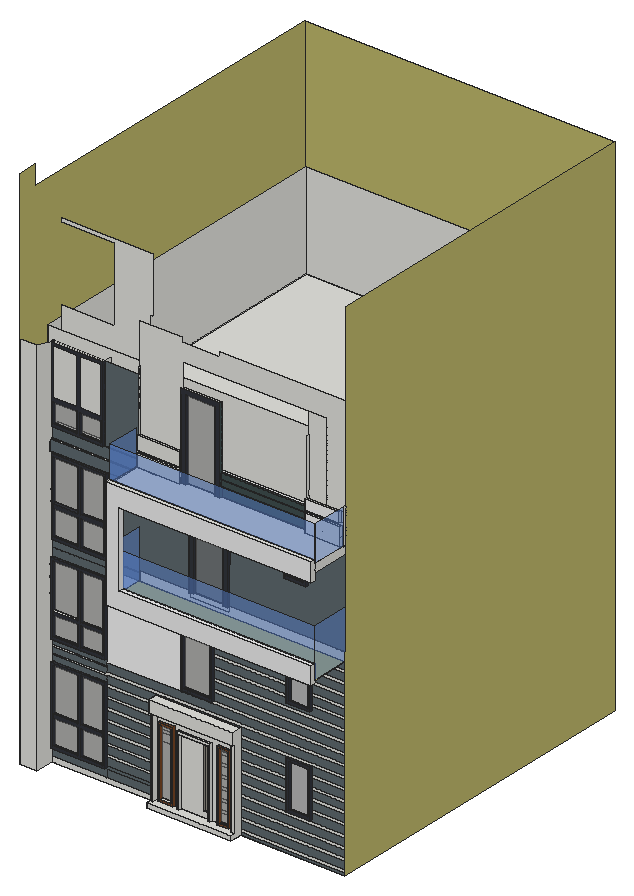
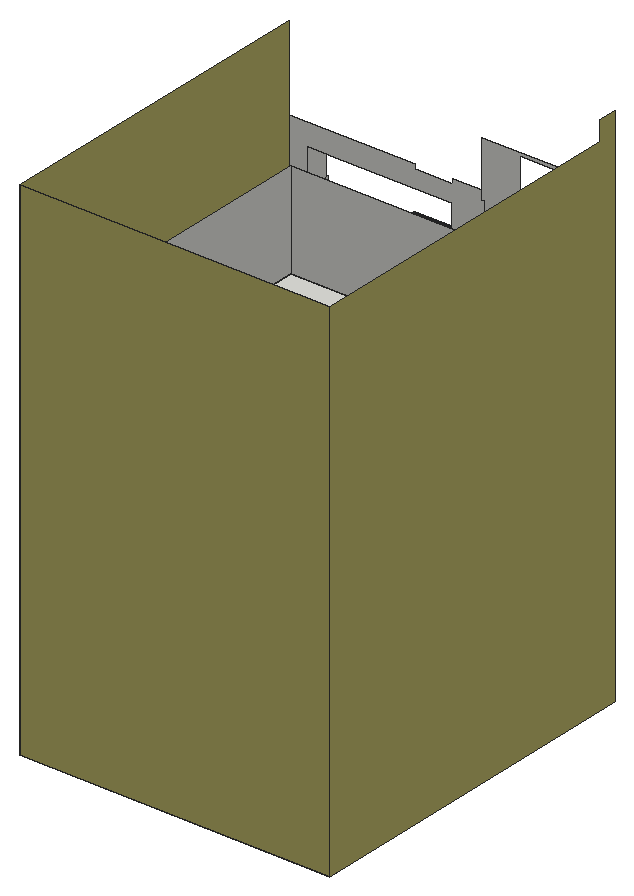
# SketchUp Ruby script. Lengths in inches.
U = 1.inch
M = Sketchup.active_model
def pt(a) = Geom::Point3d.new(a.map { |v| v * U })
def face(e, loops, mat)
  f = e.add_face(loops[0].map { |a| pt(a) })
  loops[1..].each { |l| e.add_face(l.map { |a| pt(a) }).erase! }
  f.material = f.back_material = mat if mat
  f
end
# faces: each face lists its corners as indices into pts; further lists are holes
def faces(e, pts, list, mat = nil) = list.each { |f| face(e, (f[0].is_a?(Array) ? f : [f]).map { |l| l.map { |i| pts[i] } }, mat) }
# xy, xz, yz: faces in a plane at the given z, y or x. An outline is a flat list of corners, or four numbers for a rectangle; further outlines are holes
def ring(l) = l.size == 4 ? [[l[0], l[1]], [l[2], l[1]], [l[2], l[3]], [l[0], l[3]]] : l.each_slice(2).to_a
def flat(e, list, mat, &to3) = list.each { |f| face(e, (f[0].is_a?(Array) ? f : [f]).map { |l| ring(l).map { |u, v| to3.(u, v) } }, mat) }
def xy(e, z, list, mat = nil) = flat(e, list, mat) { |x, y| [x, y, z] }
def xz(e, y, list, mat = nil) = flat(e, list, mat) { |x, z| [x, y, z] }
def yz(e, x, list, mat = nil) = flat(e, list, mat) { |y, z| [x, y, z] }
def lines(e, pts, list) = list.each { |a, b| e.add_line(pt(pts[a]), pt(pts[b])) }
# prism: a flat outline (further loops are holes) pulled along v
def prism(e, loops, v, mat = nil)
  f = face(e, loops, mat); d = Geom::Vector3d.new(v.map { |x| x * U })
  f.pushpull(f.normal.samedirection?(d) ? d.length : -d.length)
end
def box(e, o, s, mat = nil) = prism(e, [[o, [o[0] + s[0], o[1], o[2]], [o[0] + s[0], o[1] + s[1], o[2]], [o[0], o[1] + s[1], o[2]]]], [0, 0, s[2]], mat)
def at(x, y, z, deg = 0) = Geom::Transformation.translation(pt([x, y, z])) * Geom::Transformation.rotation(ORIGIN, Z_AXIS, deg.degrees)
def axes(o, x, y, z) = Geom::Transformation.new([*x, 0, *y, 0, *z, 0, *pt(o).to_a, 1])
def part(name) = M.definitions.add(name)
# library, detail: a bought-in or finely detailed component or shape, given as its bounding box
def library(name, o, s) = part(name).tap { |d| box(d.entities, o, s) }
def detail(e, o, s) = box(e.add_group.entities, o, s)
def put(e, d, t, mat = nil) = e.add_instance(d, t).tap { |i| i.material = mat if mat }
def group(e, t, mat = nil) = e.add_group.tap { |g| g.transformation = t; g.material = mat if mat }.entities
root = M.entities
M.materials.add("[0057_DarkKhaki]").color = [189, 183, 107]
M.materials.add("[0078_DarkSlateGray]").color = [63, 79, 79]
M.materials.add("[Black Pen 2]").color = [244, 244, 244]
M.materials.add("[Color M00]").color = [255, 255, 255]
M.materials.add("[Formica Graystone]").color = [149, 146, 135]
M.materials.add("[Formica Laminate Dark]").color = [50, 53, 60]
M.materials.add("[Formica Speckled Grey]").color = [94, 105, 111]
M.materials.add("[Mirror 01]").color = [185, 185, 185]
M.materials.add("[Stone Random Ashlar]").color = [240, 240, 240]
M.materials.add("[Translucent Glass Blue]").color = [100, 149, 237]
M.materials["[Translucent Glass Blue]"].alpha = 0.5
M.materials.add("[Translucent Glass Gray]").color = [128, 128, 128]
M.materials["[Translucent Glass Gray]"].alpha = 0.5
M.materials.add("[Windmill]").color = [236, 236, 236]
M.materials.add("[Wood Veneer 01]").color = [120, 70, 37]
xy(root,0,[[0,30,21.02,54],[150.64,39,255.96,51],[150.64,51,255.96,54],[[0,54,386.375,474.125],[9,63,377.375,465.125]],[9,63,377.375,465.125]])
xy(root,6.14,[[150.64,39,255.96,39,255.96,45,251.09,45,251.09,51,246.22,51,246.22,48,231.47,48,231.47,51,222.98,51,222.98,48,219.98,48,219.98,51,183.98,51,183.98,48,180.98,48,180.98,51,176.24,51,176.24,48,157.55,48,157.55,51,154.1,51,154.1,45,150.64,45],[157.55,48,176.24,51],[180.98,48,183.98,51],[219.98,48,222.98,51],[231.47,48,239.96,51],
  [239.96,48,246.22,51]])
xy(root,8.03,[[233.36,48,239.96,51],[239.96,48,244.33,51]])
xy(root,9.14,[[160.55,48,173.24,51]])
xy(root,13.03,[[212.45,51,217.33,53.3125]],"[Formica Graystone]")
xy(root,16.57,[[21.02,51,89.14,54]],"[Formica Laminate Dark]")
xy(root,19.57,[[24.02,51,55.08,54],[59.33,51,86.14,54]],"[Formica Laminate Dark]")
xy(root,48.67,[[315.34,51,344.65,54]])
xy(root,51.45,[[24.02,51,55.08,54],[59.33,51,86.14,54]],"[Formica Laminate Dark]")
xy(root,51.67,[[318.34,51,341.65,54]],"[Formica Laminate Dark]")
xy(root,55.1875,[[24.02,51,55.08,54],[59.33,51,86.14,54]],"[Formica Laminate Dark]")
xy(root,87.16,[[212.45,51,217.33,53.3125]],"[Formica Graystone]")
xy(root,90.14,[[183.98,48,219.98,51]])
xy(root,91.94,[[233.36,48,244.33,51]],"[Wood Veneer 01]")
xy(root,92.07,[[160.55,48,173.24,51]],"[Wood Veneer 01]")
xy(root,93.14,[[180.98,48,222.98,51]])
xy(root,93.82,[[231.47,48,246.22,51]],"[Wood Veneer 01]")
xy(root,95.07,[[157.55,48,176.24,51]],"[Wood Veneer 01]")
xy(root,104.875,[[150.64,42,150.64,45,154.1,45,154.1,51,251.09,51,251.09,45,255.96,45,255.96,42],[239.96,51,239.98,54]])
xy(root,105.98,[[318.34,51,341.65,54]])
xy(root,108.98,[[315.34,51,344.65,54]],"[Formica Laminate Dark]")
xy(root,109.86,[[24.02,51,55.08,54],[59.33,51,86.14,54]],"[Formica Laminate Dark]")
xy(root,112.86,[[21.02,51,89.14,54]],"[Formica Laminate Dark]")
xy(root,120,[[150.64,42,255.96,54],[9,63,377.375,465.125]])
xy(root,138.01,[[183.4,51,222.71,54]],"[Formica Laminate Dark]")
xy(root,138.82,[[21.02,51,89.14,54]],"[Formica Laminate Dark]")
xy(root,141.01,[[186.4,51,219.71,54]],"[Formica Laminate Dark]")
xy(root,141.82,[[24.02,51,55.08,54],[59.1,51,86.14,54]])
xy(root,166.59,[[24.02,51,55.08,54],[59.1,51,86.14,54]],"[Formica Laminate Dark]")
xy(root,169.86,[[24.02,51,55.08,54],[59.1,51,86.14,54]])
xy(root,169.92,[[315.34,51,344.65,54]],"[Formica Laminate Dark]")
xy(root,172.92,[[318.34,51,341.65,54]],"[Formica Laminate Dark]")
xy(root,223.89,[[186.4,51,219.71,54]],"[Formica Laminate Dark]")
xy(root,226.89,[[183.4,51,222.71,54]],"[Formica Laminate Dark]")
xy(root,227,[[24.02,51,55.08,54],[59.1,51,86.14,54]],"[Formica Laminate Dark]")
xy(root,227.23,[[318.34,51,341.65,54]],"[Formica Laminate Dark]")
xy(root,230,[[21.02,51,89.14,54]],"[Formica Laminate Dark]")
xy(root,230.23,[[315.34,51,344.65,54]],"[Formica Laminate Dark]")
xy(root,236.9375,[[130.53,0,386.375,6]])
xy(root,240,[[21.02,54,130.53,54.5],[9,63,377.375,465.125]])
xy(root,240,[[130.53,6,386.375,54]],"[0057_DarkKhaki]")
xy(root,249.57,[[21.02,54,90.08,54.5],[90.08,54,130.53,54.5]])
xy(root,249.57,[[21.02,51.5,90.08,54]],"[Formica Laminate Dark]")
xy(root,250.83,[[130.53,54,386.375,54.5]])
xy(root,252.57,[[24.02,51.5,55.55,54.5],[59.07,51.5,87.08,54.5]],"[Formica Laminate Dark]")
xy(root,258.45,[[147.37,0,386.375,6]],"[Windmill]")
xy(root,285.09,[[24.02,51.5,55.55,54.5],[59.07,51.5,87.08,54.5]],"[Formica Laminate Dark]")
xy(root,290.29,[[24.02,51.5,55.55,54.5],[59.07,51.5,87.08,54.5]],"[Formica Laminate Dark]")
xy(root,308.17,[[311.62,51.5,339,54.5]],"[Formica Laminate Dark]")
xy(root,311.17,[[314.62,51.5,336,54.5]],"[Formica Laminate Dark]")
xy(root,342.82,[[24.02,51.5,55.55,54.5],[59.07,51.5,87.08,54.5]])
xy(root,345.82,[[21.02,54,90.08,54.5,21.02,54.5]])
xy(root,345.82,[[21.02,51.5,90.08,51.5,90.08,54.5,21.02,54]],"[Formica Laminate Dark]")
xy(root,348.75,[[21.04,51,21.02,54,90.08,54.5,129.58,54.79,129.6,51.79]])
xy(root,351,[[147.37,0,386.375,6]],"[Windmill]")
xy(root,353.67,[[314.62,51.5,336,54.5]],"[Formica Laminate Dark]")
xy(root,356.67,[[311.62,51.5,339,54.5]],"[Formica Laminate Dark]")
xy(root,360,[[9,63,21.02,63,21.02,69.1875,130.53,69.1875,130.53,63,377.375,63,377.375,465.125,9,465.125],[21.02,63,90.08,69.1875],[90.08,63,130.53,69.1875]])
xy(root,360,[[130.53,6,386.375,54.5]],"[0057_DarkKhaki]")
xy(root,361.5625,[[21.04,51,129.6,51.79,129.58,54.79,90.08,54.5,21.02,54],[21.02,54,21.02,54.5,90.08,54.5]])
xy(root,362.54,[[21.02,52.875,130.53,54.5]])
xy(root,369.62,[[130.53,6,386.375,7.55],[130.53,7.55,386.375,7.55,386.375,48.5,340.48,48.5,340.48,54.5,232.02,54.5,232.02,51.5,226.02,51.5,226.02,54.5,190.02,54.5,190.02,51.5,184.02,51.5,184.02,48.5,130.53,48.5],[130.53,48.5,156.65,51.5],[156.65,48.5,184.02,51.5],[340.48,48.5,362.67,51.5],
  [362.67,48.5,383.9375,51.5],[383.9375,48.5,386.375,51.5],[130.53,51.5,184.02,54.5],[184.02,51.5,190.02,54.5],[226.02,51.5,232.02,54.5],
  [340.48,51.5,362.67,54.5],[362.67,51.5,386.375,54.5]])
xy(root,374.81,[[130.53,0,386.375,6]])
xy(root,375.92,[[21.02,51.5,86.77,52.875],[21.02,52.875,86.77,54.5],[86.77,52.875,130.53,54.5],[21.02,54.5,86.77,69.1875]])
xy(root,378.92,[[21.02,54,24.02,54.02,24.02,54.5,21.02,54.5],[53.89,54.24,57.46,54.26,57.46,54.5,53.89,54.5]])
xy(root,378.92,[[24.02,51.5,53.89,51.5,53.89,54.24,24.02,54.02],[57.46,51.5,83.77,51.5,83.77,54.45,57.46,54.26],[24.02,54.02,53.89,54.24,53.89,54.5,24.02,54.5],[57.46,54.26,83.77,54.45,83.77,54.5,57.46,54.5]],"[Formica Laminate Dark]")
xy(root,382.29,[[232.02,52.5,308.81,54.5],[308.81,52.5,340.48,54.5]])
xy(root,385.76,[[130.53,48.5,184.02,51.5]])
xy(root,389.06,[[232.02,52.5,340.48,54.5]],"[0078_DarkSlateGray]")
xy(root,389.31,[[130.53,48.5,156.65,51.5],[156.65,48.5,184.02,51.5]])
xy(root,390.91,[[232.02,52.5,343.62,54.5]])
xy(root,392.28,[[340.48,48.5,383.9375,51.5]])
xy(root,395.84,[[340.48,48.5,383.125,51.5]])
xy(root,397.68,[[232.02,52.5,343.62,54.5]],"[0078_DarkSlateGray]")
xz(root,0,[[130.53,236.9375,386.375,236.9375,386.375,258.45,147.37,258.45,147.37,351,386.375,351,386.375,374.81,130.53,374.81]],"[Windmill]")
xz(root,6,[[130.53,236.9375,386.375,240],[130.53,240,386.375,250.83],[130.53,250.83,130.53,351,147.37,351,147.37,258.45,143.18,258.45,143.18,250.83],[143.18,250.83,386.375,258.45],[130.53,351,386.375,360],
  [130.53,369.62,386.375,374.81]])
xz(root,6,[[147.37,258.45,386.375,300.91]],"[Translucent Glass Blue]")
xz(root,7.55,[[130.53,369.62,387.21,414.06]],"[Translucent Glass Blue]")
xz(root,30,[[0,0,21.02,475.71]])
xz(root,39,[[150.64,0,255.96,6.14]])
xz(root,42,[[150.64,104.875,255.96,120]])
xz(root,45,[[150.64,6.14,154.1,104.875],[251.09,6.14,255.96,104.875]])
xz(root,48,[[180.98,6.14,183.98,6.14,183.98,90.14,219.98,90.14,219.98,6.14,222.98,6.14,222.98,93.14,180.98,93.14]])
xz(root,48,[[[157.55,6.14,176.24,95.07],[160.55,9.14,173.24,92.07]],[[231.47,6.14,246.22,93.82],[233.36,8.03,244.33,91.94]]],"[Wood Veneer 01]")
xz(root,48.5,[[130.53,369.62,184.02,385.76],[130.53,389.31,184.02,405.45]])
xz(root,48.5,[[340.48,369.62,383.9375,392.28],[340.48,395.84,383.125,408.16]],"[Stone Random Ashlar]")
xz(root,51,[[180.98,3.14,222.98,6.14],[154.1,6.14,157.55,6.14,157.55,95.07,176.24,95.07,176.24,6.14,180.98,6.14,180.98,93.14,222.98,93.14,222.98,6.14,231.47,6.14,231.47,93.82,246.22,93.82,246.22,6.14,251.09,6.14,251.09,104.875,154.1,104.875],[180.98,6.14,180.98,93.14,222.98,93.14,222.98,6.14,219.98,6.14,219.98,90.14,183.98,90.14,183.98,6.14],[[183.98,6.14,219.98,90.14],[212.45,13.03,217.33,87.16]],[[231.47,6.14,246.22,93.82],[233.36,8.03,244.33,91.94]]])
xz(root,51,[[[21.02,16.57,89.14,112.86],[24.02,19.57,24.02,109.86,55.08,109.86,55.08,55.1875,24.02,55.1875,24.02,51.45,55.08,51.45,55.08,19.57],[59.33,19.57,59.33,51.45,86.14,51.45,86.14,55.1875,59.33,55.1875,59.33,109.86,86.14,109.86,86.14,19.57]],[[315.34,48.67,344.65,108.98],[318.34,51.67,341.65,105.98]],[[183.4,138.01,222.71,226.89],[186.4,141.01,219.71,223.89]],[[21.02,138.82,89.14,230],[24.02,141.82,24.02,227,55.08,227,55.08,169.86,24.02,169.86,24.02,166.59,55.08,166.59,55.08,141.82],[59.1,141.82,59.1,166.59,86.14,166.59,86.14,169.86,59.1,169.86,59.1,227,86.14,227,86.14,141.82]],[[315.34,169.92,344.65,230.23],[318.34,172.92,341.65,227.23]]],"[Formica Laminate Dark]")
xz(root,51,[[233.36,8.03,244.33,91.94],[160.55,9.14,173.24,92.07]],"[Translucent Glass Gray]")
xz(root,51.5,[[130.53,369.62,156.65,385.76],[156.65,369.62,184.02,385.76],[340.48,369.62,362.67,379.96],[362.67,369.62,383.9375,379.96],[383.9375,369.62,386.375,379.96],
  [340.48,379.96,362.67,392.28],[362.67,379.96,383.9375,392.28],[383.9375,379.96,386.375,392.28],[130.53,385.76,184.02,389.31],[130.53,389.31,156.65,405.45],
  [156.65,389.31,184.02,405.45],[340.48,392.28,386.375,395.84],[340.48,395.84,362.67,408.16],[362.67,395.84,383.125,408.16],[383.125,395.84,386.375,408.16]])
xz(root,51.5,[[[21.02,249.57,90.08,345.82],[24.02,252.57,24.02,342.82,55.55,342.82,55.55,290.29,24.02,290.29,24.02,285.09,55.55,285.09,55.55,252.57],[59.07,252.57,59.07,285.09,87.08,285.09,87.08,290.29,59.07,290.29,59.07,342.82,87.08,342.82,87.08,252.57]],[[311.62,308.17,339,356.67],[314.62,311.17,336,353.67]],[184.02,369.62,190.02,369.62,190.02,469.49,226.02,469.49,226.02,369.62,232.02,369.62,232.02,475.31,184.02,475.31],[[21.02,375.92,86.77,470.29],[24.02,378.92,24.02,467.29,53.89,467.29,53.89,408.43,24.02,408.43,24.02,403.77,53.89,403.77,53.89,378.92],[57.46,378.92,57.46,403.77,83.77,403.77,83.77,408.43,57.46,408.43,57.46,467.29,83.77,467.29,83.77,378.92]]],"[Formica Laminate Dark]")
xz(root,52.5,[[232.02,382.29,340.48,389.06],[232.02,390.91,343.62,397.68]],"[0078_DarkSlateGray]")
xz(root,52.875,[[21.02,362.54,130.53,375.92]],"[Formica Speckled Grey]")
xz(root,53.3125,[[212.45,13.03,217.33,87.16]],"[Formica Graystone]")
xz(root,54,[[21.02,0,150.64,5.81],[150.64,0,150.64,71.12,183.4,71.12,183.4,81.19,150.64,81.19,150.64,84.43,183.4,84.43,183.4,94.51,150.64,94.51,150.64,97.74,183.4,97.74,183.4,104.875,222.33,104.875,222.33,98.98,239.96,98.98,239.96,95.625,222.33,95.625,222.33,85.86,239.96,85.86,239.96,82.5,222.33,82.5,222.33,72.73,239.96,72.73,239.96,69.375,222.33,69.375,222.33,59.61,239.96,59.61,239.96,56.25,222.33,56.25,222.33,46.48,239.96,46.48,239.96,43.125,222.33,43.125,222.33,33.36,239.96,33.36,239.96,30,222.33,30,222.33,20.23,239.96,20.23,239.96,16.875,222.33,16.875,222.33,7.11,239.96,7.11,239.96,3.75,222.33,3.75,222.33,0],[222.33,0,239.96,3.75],[239.96,0,255.96,3.75],[239.96,3.75,255.96,7.11],
  [255.96,3.75,386.375,7.11],[222.33,7.11,239.96,16.875],[239.96,7.11,255.96,16.875],[[21.02,16.57,89.14,111.9],[24.02,19.57,55.08,19.57,55.08,51.45,59.33,51.45,59.33,19.57,86.14,19.57,86.14,109.86,59.33,109.86,59.33,55.1875,55.08,55.1875,55.08,109.86,24.02,109.86]],[239.96,16.875,255.96,20.23],
  [255.96,16.875,386.375,20.23],[222.33,20.23,239.96,30],[239.96,20.23,255.96,30],[89.14,28.94,150.64,31.93],[239.96,30,255.96,33.36],
  [255.96,30,386.375,33.36],[222.33,33.36,239.96,43.125],[239.96,33.36,255.96,43.125],[89.14,42.01,150.64,44.99],[239.96,43.125,255.96,46.48],
  [255.96,43.125,386.375,46.48],[222.33,46.48,239.96,56.25],[239.96,46.48,255.96,56.25],[315.34,48.67,344.65,48.67,344.65,56.25,341.65,56.25,341.65,51.67,318.34,51.67,318.34,56.25,315.34,56.25],[55.08,51.45,59.33,55.1875],
  [89.14,55.07,150.64,58.06],[239.96,56.25,255.96,59.61],[255.96,56.25,315.34,59.61],[315.34,56.25,318.34,59.61],[341.65,56.25,344.65,59.61],
  [344.65,56.25,386.375,59.61],[222.33,59.61,239.96,69.375],[239.96,59.61,255.96,69.375],[315.34,59.61,318.34,69.375],[341.65,59.61,344.65,69.375],
  [89.14,68.13,150.64,71.12],[239.96,69.375,255.96,72.73],[255.96,69.375,315.34,72.73],[315.34,69.375,318.34,72.73],[341.65,69.375,344.65,72.73],
  [344.65,69.375,386.375,72.73],[150.64,71.12,183.4,81.19],[222.33,72.73,239.96,82.5],[239.96,72.73,255.96,82.5],[315.34,72.73,318.34,82.5],
  [341.65,72.73,344.65,82.5],[89.14,81.19,150.64,84.43],[239.96,82.5,255.96,85.86],[255.96,82.5,315.34,85.86],[315.34,82.5,318.34,85.86],
  [341.65,82.5,344.65,85.86],[344.65,82.5,386.375,85.86],[150.64,84.43,183.4,94.51],[222.33,85.86,239.96,95.625],[239.96,85.86,255.96,95.625],
  [315.34,85.86,318.34,95.625],[341.65,85.86,344.65,95.625],[89.14,94.51,150.64,97.74],[239.96,95.625,255.96,98.98],[255.96,95.625,315.34,98.98],
  [315.34,95.625,318.34,98.98],[341.65,95.625,344.65,98.98],[344.65,95.625,386.375,98.98],[150.64,97.74,183.4,104.875],[222.33,98.98,239.96,104.875],
  [239.96,98.98,255.96,104.875],[315.34,98.98,318.34,98.98,318.34,105.98,341.65,105.98,341.65,98.98,344.65,98.98,344.65,108.75,315.34,108.75],[150.64,104.875,183.4,107.82],[222.33,104.875,239.98,108.75],[239.98,104.875,255.96,108.75],
  [89.14,107.82,150.64,111.06],[239.98,108.75,255.96,112.11],[255.96,108.75,315.34,108.75,315.34,108.98,344.65,108.98,344.65,108.75,386.375,108.75,386.375,112.11,255.96,112.11],[315.34,108.75,344.65,108.98],[150.64,111.06,183.4,120],
  [21.02,111.9,89.14,112.86],[222.33,112.11,239.98,120],[239.98,112.11,255.96,120],[21.02,119.88,89.14,119.88,89.14,121.13,183.4,121.13,222.33,121.875,386.375,121.875,386.375,125.23,222.33,125.23,183.4,124.37,89.14,124.37,89.14,121.34,21.02,121.34],[21.02,129.32,89.14,130.84],
  [183.26,134.44,183.4,134.44,222.33,135,386.375,135,386.375,138.36,222.71,138.36,222.71,138.01,183.4,138.01,183.4,137.68,183.26,137.68],[183.26,137.68,183.4,147.76],[[183.4,138.01,183.4,226.89,222.71,226.89,222.71,226.875,222.33,226.875,222.33,217.11,222.71,217.11,222.71,213.75,222.33,213.75,222.33,203.98,222.71,203.98,222.71,200.625,222.33,200.625,222.33,190.86,222.71,190.86,222.71,187.5,222.33,187.5,222.33,177.73,222.71,177.73,222.71,174.375,222.33,174.375,222.33,164.61,222.71,164.61,222.71,161.25,222.33,161.25,222.33,151.48,222.71,151.48,222.71,148.125,222.33,148.125,222.33,138.36,222.71,138.36,222.71,138.01],[186.4,141.01,219.71,223.89]],[222.33,138.36,222.71,148.125],[[21.02,138.82,89.14,230],[24.02,141.82,55.08,141.82,55.08,166.59,59.1,166.59,59.1,141.82,86.14,141.82,86.14,227,59.1,227,59.1,169.86,55.08,169.86,55.08,227,24.02,227]],
  [183.26,147.76,183.4,150.99],[222.71,148.125,386.375,151.48],[183.26,150.99,183.4,161.07],[222.33,151.48,222.71,161.25],[183.26,161.07,183.4,164.31],
  [222.71,161.25,386.375,164.61],[183.26,164.31,183.4,174.38],[222.33,164.61,222.71,174.375],[55.08,166.59,59.1,169.86],[315.34,169.92,344.65,169.92,344.65,174.375,341.65,174.375,341.65,172.92,318.34,172.92,318.34,174.375,315.34,174.375],
  [222.71,174.375,315.34,177.73],[315.34,174.375,318.34,177.73],[341.65,174.375,344.65,177.73],[344.65,174.375,386.375,177.73],[183.26,174.38,183.4,177.62],
  [183.26,177.62,183.4,187.69],[222.33,177.73,222.71,187.5],[315.34,177.73,318.34,187.5],[341.65,177.73,344.65,187.5],[222.71,187.5,315.34,190.86],
  [315.34,187.5,318.34,190.86],[341.65,187.5,344.65,190.86],[344.65,187.5,386.375,190.86],[183.26,187.69,183.4,190.93],[222.33,190.86,222.71,200.625],
  [315.34,190.86,318.34,200.625],[341.65,190.86,344.65,200.625],[183.26,190.93,183.4,201.01],[222.71,200.625,315.34,203.98],[315.34,200.625,318.34,203.98],
  [341.65,200.625,344.65,203.98],[344.65,200.625,386.375,203.98],[183.26,201.01,183.4,204.24],[222.33,203.98,222.71,213.75],[315.34,203.98,318.34,213.75],
  [341.65,203.98,344.65,213.75],[183.26,204.24,183.4,214.32],[222.71,213.75,315.34,217.11],[315.34,213.75,318.34,217.11],[341.65,213.75,344.65,217.11],
  [344.65,213.75,386.375,217.11],[183.26,214.32,183.4,216.62],[183.26,216.62,183.4,226.69],[222.33,217.11,222.71,226.875],[315.34,217.11,318.34,226.875],
  [341.65,217.11,344.65,226.875],[183.26,226.69,183.4,226.69,183.4,226.89,222.71,226.89,222.71,226.875,315.34,226.875,315.34,230.23,183.26,230.23],[315.34,226.875,315.34,230.23,344.65,230.23,344.65,226.875,341.65,226.875,341.65,227.23,318.34,227.23,318.34,226.875],[318.34,226.875,341.65,227.23],[344.65,226.875,386.375,230.23],
  [21.02,230,89.14,230.23],[130.53,240,386.375,250.83]])
xz(root,54,[[89.14,134.44,183.26,240]],"[Black Pen 2]")
xz(root,54,[[255.96,0,386.375,3.75],[21.02,5.81,89.14,5.81,89.14,15.88,150.64,15.88,150.64,18.87,89.14,18.87,89.14,16.57,21.02,16.57],[89.14,5.81,150.64,15.88],[255.96,7.11,386.375,16.875],[89.14,18.87,150.64,28.94],
  [255.96,20.23,386.375,30],[89.14,31.93,150.64,42.01],[255.96,33.36,386.375,43.125],[89.14,44.99,150.64,55.07],[255.96,46.48,386.375,46.48,386.375,56.25,344.65,56.25,344.65,48.67,315.34,48.67,315.34,56.25,255.96,56.25],
  [89.14,58.06,150.64,68.13],[255.96,59.61,315.34,69.375],[344.65,59.61,386.375,69.375],[89.14,71.12,150.64,81.19],[255.96,72.73,315.34,82.5],
  [344.65,72.73,386.375,82.5],[89.14,84.43,150.64,94.51],[255.96,85.86,315.34,95.625],[344.65,85.86,386.375,95.625],[89.14,97.74,150.64,107.82],
  [255.96,98.98,315.34,108.75],[344.65,98.98,386.375,108.75],[89.14,111.06,150.64,111.06,150.64,120,255.96,120,255.96,112.11,386.375,112.11,386.375,121.875,222.33,121.875,183.4,121.13,89.14,121.13],[21.02,112.86,89.14,119.88],[21.02,121.34,89.14,129.32],
  [89.14,124.37,183.4,124.37,222.33,125.23,386.375,125.23,386.375,135,222.33,135,183.4,134.44,89.14,134.44],[21.02,130.84,89.14,138.82],[222.71,138.36,386.375,148.125],[222.71,151.48,386.375,161.25],[222.71,164.61,386.375,164.61,386.375,174.375,344.65,174.375,344.65,169.92,315.34,169.92,315.34,174.375,222.71,174.375],
  [222.71,177.73,315.34,187.5],[344.65,177.73,386.375,187.5],[222.71,190.86,315.34,200.625],[344.65,190.86,386.375,200.625],[222.71,203.98,315.34,213.75],
  [344.65,203.98,386.375,213.75],[222.71,217.11,315.34,226.875],[344.65,217.11,386.375,226.875],[21.02,230.23,89.14,240],[183.26,230.23,386.375,240],
  [21.02,240,130.53,249.57]],"[Formica Speckled Grey]")
xz(root,54,[[318.34,51.67,341.65,105.98],[318.34,172.92,341.65,226.875]],"[Mirror 01]")
xz(root,54,[[24.02,19.57,55.08,51.45],[59.33,19.57,86.14,51.45],[24.02,55.1875,55.08,109.86],[59.33,55.1875,86.14,109.86],[186.4,141.01,219.71,223.89],
  [24.02,141.82,55.08,166.59],[59.1,141.82,86.14,166.59],[24.02,169.86,55.08,227],[59.1,169.86,86.14,227]],"[Translucent Glass Gray]")
xz(root,54.5,[[21.02,240,90.08,249.57],[90.08,240,130.53,249.57],[[21.02,249.57,90.08,345.82],[24.02,252.57,55.55,252.57,55.55,285.09,59.07,285.09,59.07,252.57,87.08,252.57,87.08,342.82,59.07,342.82,59.07,290.29,55.55,290.29,55.55,342.82,24.02,342.82]],[55.55,285.09,59.07,290.29],[[311.62,308.17,339,356.67],[314.62,311.17,336,353.67]],
  [130.53,360,130.53,369.62,184.02,369.62,184.02,363.62,232.02,363.62,232.02,369.62,386.375,369.62,386.375,360],[184.02,363.62,232.02,369.62],[130.53,369.62,130.53,530.7,181.91,530.7,181.91,524.72,229.91,524.72,229.91,530.72,386.375,530.72,386.375,369.62,362.67,369.62,362.67,503.41,184.02,503.41,184.02,369.62],[184.02,369.62,184.02,475.31,232.02,475.31,232.02,369.62,226.02,369.62,226.02,469.49,190.02,469.49,190.02,369.62],[340.48,369.62,340.48,390.91,343.62,390.91,343.62,397.68,340.48,397.68,340.48,417.77,340.5,417.77,340.5,476.58,340.48,476.58,340.48,503.41,362.67,503.41,362.67,369.62],
  [21.02,375.92,86.77,378.92],[232.02,382.29,308.81,389.06],[308.81,382.29,340.48,389.06],[232.02,390.91,308.81,397.68],[308.81,390.91,340.48,397.68],
  [340.48,390.91,343.62,397.68]])
xz(root,54.5,[[232.02,369.62,340.48,382.29]],"[0078_DarkSlateGray]")
xz(root,54.5,[[232.02,389.06,340.48,390.91],[232.02,397.68,340.48,399.54]],"[Color M00]")
xz(root,54.5,[[[90.08,249.57,130.53,249.57,130.53,250.83,386.375,250.83,386.375,360,130.53,360,130.53,362.54,21.02,362.54,21.02,345.82,90.08,345.82],[311.62,308.17,339,356.67]],[86.77,375.92,130.53,375.92,130.53,470.57,21.02,470.57,21.02,470.29,86.77,470.29]],"[Formica Speckled Grey]")
xz(root,54.5,[[314.62,311.17,336,353.67]],"[Mirror 01]")
xz(root,54.5,[[24.02,252.57,55.55,285.09],[59.07,252.57,87.08,285.09],[24.02,290.29,55.55,342.82],[59.07,290.29,87.08,342.82],[190.02,369.62,226.02,469.49],
  [24.02,378.92,53.89,403.77],[57.46,378.92,83.77,403.77]],"[Translucent Glass Gray]")
xz(root,63,[[9,0,377.375,120],[9,120,377.375,240],[9,240,377.375,360],[9,360,377.375,480]])
xz(root,69.1875,[[21.02,360,21.02,375.92,86.77,375.92,86.77,470.29,21.02,470.29,21.02,503.32,87.52,503.32,87.52,596.25,21.02,596.25,21.02,600,134.96,600,134.96,530.72,130.53,530.72,130.53,360]])
xz(root,465.125,[[9,0,377.375,120],[9,120,377.375,240],[9,240,377.375,360],[9,360,377.375,480]])
xz(root,474.125,[[0,0,386.375,636]],"[0057_DarkKhaki]")
yz(root,0,[[30,0,30,660,54,660,54,636,474.125,636,474.125,0]],"[0057_DarkKhaki]")
yz(root,9,[[63,0,465.125,120],[63,120,465.125,240],[63,240,465.125,360],[63,360,465.125,480]])
yz(root,21.02,[[30,0,54,0,54,16.57,51,16.57,51,112.86,54,112.86,54,138.82,51,138.82,51,230,54,230,54,249.57,51.5,249.57,51.5,345.82,54,345.82,54,362.54,52.875,362.54,52.875,375.92,51.5,375.92,51.5,470.29,30,475.71],[51,16.57,54,111.9],[51,111.9,54,112.86],[51,138.82,54,230],[54,240,54.5,249.57],
  [51.5,249.57,54,345.82],[54,249.57,54.5,345.82],[54,345.82,54.5,360],[54,360,54.5,361.5625],[54.5,360,69.1875,375.92],
  [54,361.5625,54.5,362.54],[52.875,362.54,54,375.92],[54,362.54,54.5,375.92],[51.5,375.92,54,378.92],[54,375.92,54.5,378.92],
  [51.5,378.92,54,470.29],[54,378.92,54.5,470.29]])
yz(root,24.02,[[51,51.45,54,55.1875],[51,166.59,54,169.86],[51.5,285.09,54.5,290.29]])
yz(root,24.02,[[51,19.57,54,51.45],[51,55.1875,54,109.86],[51,141.82,54,166.59],[51,169.86,54,227],[51.5,252.57,54.5,285.09],
  [51.5,290.29,54.5,342.82],[51.5,378.92,54.5,403.77]],"[Formica Laminate Dark]")
yz(root,53.89,[[51.5,378.92,54.5,403.77]],"[Formica Laminate Dark]")
yz(root,55.08,[[51,141.82,54,166.59],[51,169.86,54,227]])
yz(root,55.08,[[51,19.57,54,51.45],[51,55.1875,54,109.86]],"[Formica Laminate Dark]")
yz(root,55.55,[[51.5,252.57,54.5,285.09],[51.5,290.29,54.5,342.82]],"[Formica Laminate Dark]")
yz(root,57.46,[[51.5,378.92,54.5,403.77]],"[Formica Laminate Dark]")
yz(root,59.07,[[51.5,252.57,54.5,285.09],[51.5,290.29,54.5,342.82]],"[Formica Laminate Dark]")
yz(root,59.1,[[51,141.82,54,166.59],[51,169.86,54,227]],"[Formica Laminate Dark]")
yz(root,59.33,[[51,19.57,54,51.45],[51,55.1875,54,109.86]],"[Formica Laminate Dark]")
yz(root,83.77,[[51.5,378.92,54.5,403.77]],"[Formica Laminate Dark]")
yz(root,86.14,[[51,51.45,54,55.1875],[51,141.82,54,166.59],[51,166.59,54,169.86],[51,169.86,54,227]])
yz(root,86.14,[[51,19.57,54,51.45],[51,55.1875,54,109.86]],"[Formica Laminate Dark]")
yz(root,86.77,[[54.5,375.92,69.1875,470.29]])
yz(root,86.77,[[51.5,375.92,54.5,470.29]],"[Formica Laminate Dark]")
yz(root,87.08,[[51.5,285.09,54.5,290.29]])
yz(root,87.08,[[51.5,252.57,54.5,285.09],[51.5,290.29,54.5,342.82]],"[Formica Laminate Dark]")
yz(root,89.14,[[51,16.57,54,112.86],[51,138.82,54,230]],"[Formica Laminate Dark]")
yz(root,90.08,[[51.5,249.57,54.5,345.82]],"[Formica Laminate Dark]")
yz(root,130.53,[[0,236.9375,0,374.81,6,374.81,6,369.62,52.875,369.62,52.875,362.54,54.5,362.54,54.5,360,6,360,6,236.9375],[54,240,54.5,249.57],[54,249.57,54.5,250.83],[54.5,360,69.1875,369.62],[52.875,362.54,54.5,369.62],
  [48.5,369.62,51.5,385.76],[51.5,369.62,51.5,480,52.5,480,52.5,479.5,54.5,479.5,54.5,477.57,52.5,477.57,52.5,470.57,54.5,470.57,54.5,375.92,52.875,375.92,52.875,369.62],[52.875,369.62,54.5,375.92],[54.5,369.62,69.1875,480],[48.5,385.76,51.5,389.31],
  [48.5,389.31,51.5,405.45]])
yz(root,130.53,[[6,240,54,300.91],[7.55,369.62,48.5,414.06]],"[Translucent Glass Blue]")
yz(root,147.37,[[0,258.45,6,351]],"[Windmill]")
yz(root,150.64,[[39,0,39,6.14,45,6.14,45,104.875,42,104.875,42,120,54,120,54,0]])
yz(root,154.1,[[45,6.14,51,104.875]])
yz(root,157.55,[[48,6.14,51,95.07]],"[Wood Veneer 01]")
yz(root,160.55,[[48,9.14,51,92.07]],"[Wood Veneer 01]")
yz(root,173.24,[[48,9.14,51,92.07]],"[Wood Veneer 01]")
yz(root,176.24,[[48,6.14,51,95.07]],"[Wood Veneer 01]")
yz(root,180.98,[[48,6.14,51,93.14]])
yz(root,183.4,[[51,138.01,54,226.89]],"[Formica Laminate Dark]")
yz(root,183.98,[[48,6.14,51,90.14]])
yz(root,184.02,[[48.5,369.62,51.5,385.76],[51.5,369.62,54.5,468.06],[48.5,389.31,51.5,405.45]])
yz(root,186.4,[[51,141.01,54,223.89]],"[Formica Laminate Dark]")
yz(root,190.02,[[51.5,369.62,54.5,469.49]],"[Formica Laminate Dark]")
yz(root,193.84,[[54,250.83,51,250.84,51.45,340.84,54.45,340.83]],"[Formica Laminate Dark]")
yz(root,199.84,[[54.8125,250.82,54,250.83,54.42,334.83,55.24,334.82]])
yz(root,199.84,[[54,250.83,54.42,334.83,51.42,334.84,51,250.84]],"[Formica Laminate Dark]")
yz(root,212.45,[[51,13.03,53.3125,87.16]],"[Formica Graystone]")
yz(root,217.33,[[51,13.03,53.3125,87.16]],"[Formica Graystone]")
yz(root,219.71,[[51,141.01,54,223.89]],"[Formica Laminate Dark]")
yz(root,219.98,[[48,6.14,51,90.14]])
yz(root,222.71,[[51,138.01,54,226.89]],"[Formica Laminate Dark]")
yz(root,222.98,[[48,6.14,51,93.14]])
yz(root,226.02,[[51.5,369.62,54.5,469.49]],"[Formica Laminate Dark]")
yz(root,231.47,[[48,6.14,51,93.82]],"[Wood Veneer 01]")
yz(root,232.02,[[52.5,382.29,54.5,389.06],[52.5,390.91,54.5,397.68]])
yz(root,232.02,[[51.5,369.62,54.5,369.62,54.5,382.29,52.5,382.29,52.5,389.06,54.5,389.06,54.5,390.91,52.5,390.91,52.5,397.68,54.5,397.68,54.5,399.54,52.5,399.54,52.5,406.31,54.5,406.31,54.5,408.16,52.5,408.16,52.5,414.93,54.5,414.93,54.5,416.79,52.5,416.79,52.5,423.56,54.5,423.56,54.5,425.41,52.5,425.41,52.5,432.18,54.5,432.18,54.5,434.04,52.5,434.04,52.5,440.81,54.5,440.81,54.5,442.66,52.5,442.66,52.5,449.43,54.5,449.43,54.5,451.29,52.5,451.29,52.5,458.06,54.5,458.06,54.5,459.91,52.5,459.91,52.5,466.68,54.5,466.68,54.5,468.54,52.5,468.54,52.5,475.31,51.5,475.31]],"[0078_DarkSlateGray]")
yz(root,233.36,[[48,8.03,51,91.94]],"[Wood Veneer 01]")
yz(root,235.84,[[54.8125,250.82,55.24,334.82,54.42,334.83,54,250.83]])
yz(root,235.84,[[54,250.83,51,250.84,51.42,334.84,54.42,334.83]],"[Formica Laminate Dark]")
yz(root,241.84,[[54,250.83,54.45,340.83,51.45,340.84,51,250.84]],"[Formica Laminate Dark]")
yz(root,244.33,[[48,8.03,51,91.94]],"[Wood Veneer 01]")
yz(root,246.22,[[48,6.14,51,93.82]],"[Wood Veneer 01]")
yz(root,251.09,[[45,6.14,51,104.875]])
yz(root,255.96,[[39,0,54,0,54,120,42,120,42,104.875,45,104.875,45,6.14,39,6.14]])
yz(root,311.62,[[51.5,308.17,54.5,356.67]],"[Formica Laminate Dark]")
yz(root,314.62,[[51.5,311.17,54.5,353.67]],"[Formica Laminate Dark]")
yz(root,315.34,[[51,48.67,54,108.98],[51,169.92,54,230.23]],"[Formica Laminate Dark]")
yz(root,318.34,[[51,51.67,54,105.98],[51,172.92,54,227.23]],"[Formica Laminate Dark]")
yz(root,336,[[51.5,311.17,54.5,353.67]],"[Formica Laminate Dark]")
yz(root,339,[[51.5,308.17,54.5,356.67]],"[Formica Laminate Dark]")
yz(root,340.48,[[48.5,369.62,51.5,379.96],[51.5,369.62,51.5,476.6,54.5,476.6,54.5,414.93,52.5,414.93,52.5,408.16,54.5,408.16,54.5,406.31,52.5,406.31,52.5,399.54,54.5,399.54,54.5,389.06,52.5,389.06,52.5,382.29,54.5,382.29,54.5,369.62],[48.5,379.96,51.5,392.28],[48.5,395.84,51.5,408.16]])
yz(root,341.65,[[51,51.67,54,105.98],[51,172.92,54,227.23]],"[Formica Laminate Dark]")
yz(root,343.62,[[52.5,390.91,54.5,397.68]])
yz(root,344.65,[[51,48.67,54,108.98],[51,169.92,54,230.23]],"[Formica Laminate Dark]")
yz(root,377.375,[[63,0,465.125,120],[63,120,465.125,240],[63,240,465.125,360],[63,360,465.125,480]])
yz(root,383.125,[[48.5,395.84,51.5,408.16]])
yz(root,383.9375,[[48.5,369.62,51.5,379.96],[48.5,379.96,51.5,392.28]])
yz(root,386.375,[[0,236.9375,6,258.45],[0,351,6,374.81],[6,360,54.5,369.62],[51.5,369.62,54.5,414.3]])
yz(root,386.375,[[54,0,474.125,0,474.125,636,54.5,636,54.5,250.83,54,250.83]],"[0057_DarkKhaki]")
yz(root,386.375,[[6,240,54,240,54,250.83,54.5,250.83,54.5,300.91,6,300.91],[6,369.62,51.5,414.3]],"[Translucent Glass Blue]")
p = [[241.84,53.97,244.83],[241.84,54,250.83],[235.84,54,250.83],[199.84,54,250.83],[193.84,54,250.83],[193.84,53.97,244.83],
  [199.84,51,250.84],[193.84,51,250.84],[241.84,51,250.84],[241.84,51.45,340.84],[193.84,51.45,340.84],[199.84,51.42,334.84],
  [235.84,51.42,334.84],[235.84,51,250.84],[241.84,54.45,340.83],[235.84,54.42,334.83],[199.84,54.42,334.83],[193.84,54.45,340.83],
  [199.84,54.8125,250.82],[235.84,54.8125,250.82],[199.84,55.24,334.82],[235.84,55.24,334.82],[21.04,51,361.5625],[21.04,51,348.75],
  [129.6,51.79,348.75],[129.6,51.79,361.5625],[21.02,54,348.75],[21.02,54,361.5625],[21.02,54,360],[129.58,54.79,348.75],
  [129.58,54.79,360],[129.58,54.79,361.5625],[90.08,54.5,361.5625],[90.08,54.5,360],[90.08,54.5,348.75],[239.96,51,0],
  [239.96,51,6.14],[386.375,7.55,413.84],[386.375,7.55,369.62],[362.67,51.5,379.96],[362.67,48.5,379.96],[90.08,63,360]]
faces(root,p,[[0,1,2,3,4,5],[4,3,6,7],[2,1,8,13],[14,1,2,15,16,3,4,17],[2,3,18,19],[18,20,21,19],[16,15,21,20],[26,23,22,27,28],
  [29,30,31,25,24],[26,28,27,32,33,34],[34,33,30,29],[33,32,31,30]])
faces(root,p,[[8,9,10,7,6,11,12,13],[16,15,12,11],[14,17,10,9]],"[Formica Laminate Dark]")
faces(root,p,[[16,3,2,15]],"[Translucent Glass Gray]")
faces(root,p,[[22,23,24,25]],"[Formica Speckled Grey]")
lines(root,p,[[35,36],[37,38],[39,40],[33,41]])
